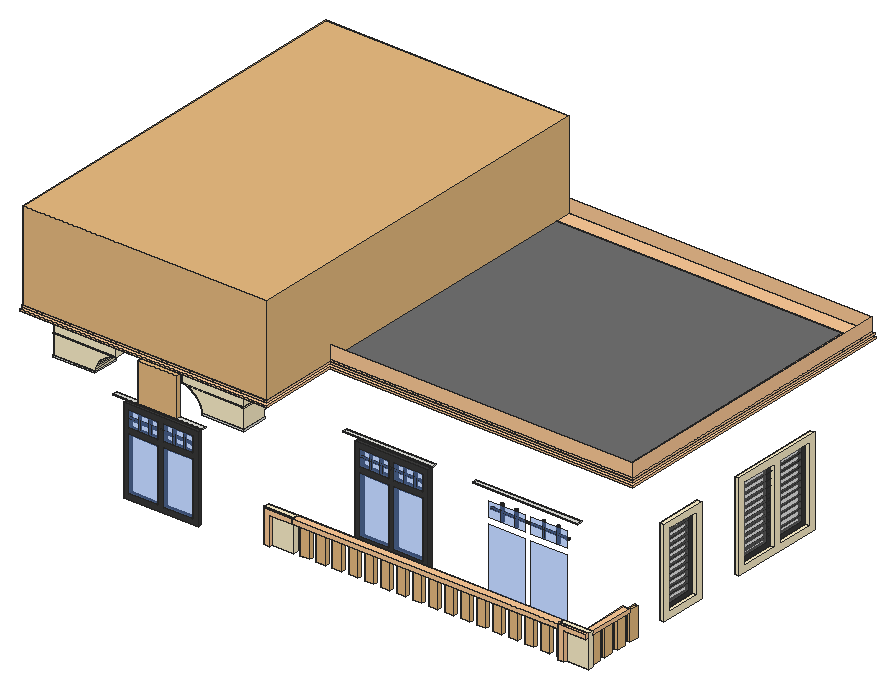
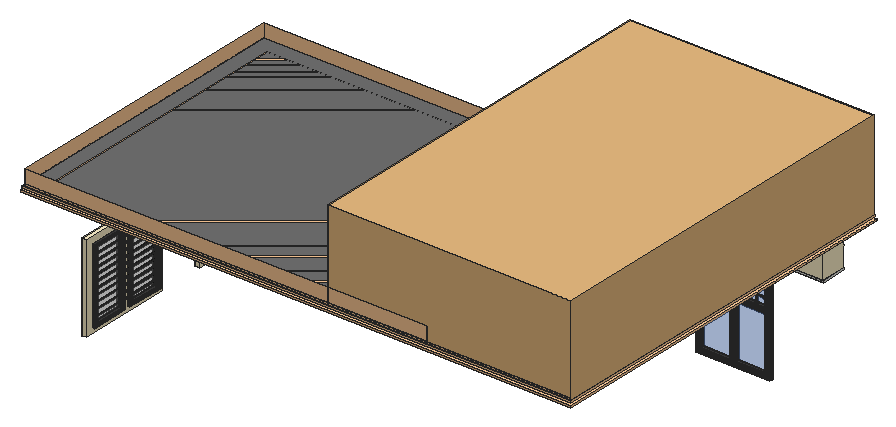
# SketchUp Ruby script. Lengths in inches.
U = 1.inch
M = Sketchup.active_model
def pt(a) = Geom::Point3d.new(a.map { |v| v * U })
def face(e, loops, mat)
  f = e.add_face(loops[0].map { |a| pt(a) })
  loops[1..].each { |l| e.add_face(l.map { |a| pt(a) }).erase! }
  f.material = f.back_material = mat if mat
  f
end
# faces: each face lists its corners as indices into pts; further lists are holes
def faces(e, pts, list, mat = nil) = list.each { |f| face(e, (f[0].is_a?(Array) ? f : [f]).map { |l| l.map { |i| pts[i] } }, mat) }
# xy, xz, yz: faces in a plane at the given z, y or x. An outline is a flat list of corners, or four numbers for a rectangle; further outlines are holes
def ring(l) = l.size == 4 ? [[l[0], l[1]], [l[2], l[1]], [l[2], l[3]], [l[0], l[3]]] : l.each_slice(2).to_a
def flat(e, list, mat, &to3) = list.each { |f| face(e, (f[0].is_a?(Array) ? f : [f]).map { |l| ring(l).map { |u, v| to3.(u, v) } }, mat) }
def xy(e, z, list, mat = nil) = flat(e, list, mat) { |x, y| [x, y, z] }
def xz(e, y, list, mat = nil) = flat(e, list, mat) { |x, z| [x, y, z] }
def yz(e, x, list, mat = nil) = flat(e, list, mat) { |y, z| [x, y, z] }
def lines(e, pts, list) = list.each { |a, b| e.add_line(pt(pts[a]), pt(pts[b])) }
# prism: a flat outline (further loops are holes) pulled along v
def prism(e, loops, v, mat = nil)
  f = face(e, loops, mat); d = Geom::Vector3d.new(v.map { |x| x * U })
  f.pushpull(f.normal.samedirection?(d) ? d.length : -d.length)
end
def box(e, o, s, mat = nil) = prism(e, [[o, [o[0] + s[0], o[1], o[2]], [o[0] + s[0], o[1] + s[1], o[2]], [o[0], o[1] + s[1], o[2]]]], [0, 0, s[2]], mat)
def at(x, y, z, deg = 0) = Geom::Transformation.translation(pt([x, y, z])) * Geom::Transformation.rotation(ORIGIN, Z_AXIS, deg.degrees)
def axes(o, x, y, z) = Geom::Transformation.new([*x, 0, *y, 0, *z, 0, *pt(o).to_a, 1])
def part(name) = M.definitions.add(name)
# library, detail: a bought-in or finely detailed component or shape, given as its bounding box
def library(name, o, s) = part(name).tap { |d| box(d.entities, o, s) }
def detail(e, o, s) = box(e.add_group.entities, o, s)
def put(e, d, t, mat = nil) = e.add_instance(d, t).tap { |i| i.material = mat if mat }
def group(e, t, mat = nil) = e.add_group.tap { |g| g.transformation = t; g.material = mat if mat }.entities
root = M.entities
M.materials.add("[Color C02]").color = [255, 204, 153]
M.materials.add("[Color D01]").color = [255, 242, 204]
M.materials.add("[Color M05]").color = [114, 114, 114]
M.materials.add("[Color M07]").color = [58, 58, 58]
M.materials.add("[Color M08]").color = [30, 30, 30]
M.materials.add("[Translucent Glass Blue]").color = [100, 149, 237]
M.materials["[Translucent Glass Blue]"].alpha = 0.5
M.materials.add("[Translucent Glass Gray]").color = [128, 128, 128]
M.materials["[Translucent Glass Gray]"].alpha = 0.5
c1 = part("Group\#116")
box(c1.entities,[0,0,0],[33.28,6,36])
c2 = part("Group\#117")
xy(c2.entities,0,[[0,0,7.19,3]])
xy(c2.entities,31.08,[[7.19,0,31.28,3]])
xy(c2.entities,36,[[0,0,7.19,3],[7.19,0,31.28,3]])
xz(c2.entities,0,[[0,0,7.19,0,7.19,31.08,31.28,31.08,31.28,36,0,36]])
xz(c2.entities,3,[[0,0,7.19,36],[7.19,31.08,31.28,36]])
yz(c2.entities,0,[[0,0,3,36]])
yz(c2.entities,7.19,[[0,0,3,31.08]])
yz(c2.entities,31.28,[[0,31.08,3,36]])
c3 = library("Group\#119",[0,0,0],[10.6875,3.6875,32.1875])
c4 = part("Group\#73")
prism(c4.entities,[[[0.41,0,0.11],[0.6,0,0.03],[0.8125,0,0],[1.02,0,0.03],[1.22,0,0.11],[1.39,0,0.24],[1.52,0,0.41],[1.6,0,0.6],[1.625,0,0.8125],[1.6,0,1.02],[1.52,0,1.22],[1.39,0,1.39],[1.22,0,1.52],[1.02,0,1.6],[0.8125,0,1.625],[0.6,0,1.6],[0.41,0,1.52],[0.24,0,1.39],[0.11,0,1.22],[0.03,0,1.02],[0,0,0.8125],[0.03,0,0.6],[0.11,0,0.41],[0.24,0,0.24]]],[0,83.52,0])
c5 = part("Group\#71")
prism(c5.entities,[[[1.26,30.72,0.03],[1,30.72,0],[0.74,30.72,0.03],[0.5,30.72,0.13],[0.29,30.72,0.29],[0.13,30.72,0.5],[0.03,30.72,0.74],[0,30.72,1],[0.03,30.72,1.26],[0.13,30.72,1.5],[0.29,30.72,1.71],[0.5,30.72,1.87],[0.74,30.72,1.97],[1,30.72,2],[1.26,30.72,1.97],[1.5,30.72,1.87],[1.71,30.72,1.71],[1.87,30.72,1.5],[1.97,30.72,1.26],[2,30.72,1],[1.97,30.72,0.74],[1.87,30.72,0.5],[1.71,30.72,0.29],[1.5,30.72,0.13]]],[0,-30.72,0])
c6 = part("Group\#104")
box(c6.entities,[-1,-1,0],[47.74,29,1.9375])
c7 = library("Group\#113",[-1.05,-1.3,0],[273.09,424.42,99.7])
xy(root,387.9375,[[446.12,288.64,786.76,619.71]])
xy(root,391.9375,[[338.37,286.64,788.76,621.71]],"[Color M05]")
xz(root,286.64,[[338.37,391.9375,788.76,407.09]],"[Color C02]")
xz(root,621.71,[[338.37,391.9375,788.76,407.09]],"[Color C02]")
yz(root,338.37,[[286.64,391.9375,621.71,407.09]],"[Color M05]")
yz(root,788.76,[[286.64,391.9375,621.71,407.09]],"[Color C02]")
g1 = group(root,at(660.76,304.14,204),"[Translucent Glass Blue]")
xz(g1,0,[[0,0,41,72]])
g2 = group(root,at(613.76,304.14,204),"[Translucent Glass Blue]")
xz(g2,0,[[0,0,41,72]])
g3 = group(root,at(462.04,304.64,206),"[Color M07]")
prism(g3,[[[82.52,5,0],[0,5,0],[0,5,100],[82.52,5,100]],[[6,5,6],[38.26,5,6],[38.26,5,70],[6,5,70]],[[44.26,5,70],[44.26,5,6],[76.52,5,6],[76.52,5,70]],[[6,5,76],[38.26,5,76],[38.26,5,94],[6,5,94]],[[44.26,5,76],[76.52,5,76],[76.52,5,94],[44.26,5,94]]],[0,-5,0])
g4 = group(root,at(260.38,232.64,210),"[Color M07]")
prism(g4,[[[0,0,96],[0,0,0],[84,0,0],[84,0,96]],[[6,0,66],[39,0,66],[39,0,6],[6,0,6]],[[78,0,66],[78,0,6],[45,0,6],[45,0,66]],[[78,0,72],[45,0,72],[45,0,90],[78,0,90]],[[6,0,72],[6,0,90],[39,0,90],[39,0,72]]],[0,4,0])
put(root,c1,at(406.12,247.64,210),"[Color D01]")
put(root,c2,at(408.12,244.64,210),"[Color C02]")
put(root,c1,at(737.48,247.64,210),"[Color D01]")
put(root,c2,at(738.31,244.64,210),"[Color C02]")
put(root,c3,at(445.87,248.72,210),"[Color D01]")
put(root,c3,at(463.87,248.72,210),"[Color D01]")
put(root,c3,at(481.87,248.72,210),"[Color D01]")
put(root,c3,at(499.87,248.72,210),"[Color D01]")
put(root,c3,at(517.87,248.72,210),"[Color D01]")
put(root,c3,at(535.87,248.72,210),"[Color D01]")
put(root,c3,at(553.87,248.72,210),"[Color D01]")
put(root,c3,at(571.87,248.72,210),"[Color D01]")
put(root,c3,at(589.87,248.72,210),"[Color D01]")
put(root,c3,at(607.87,248.72,210),"[Color D01]")
put(root,c3,at(625.87,248.72,210),"[Color D01]")
put(root,c3,at(643.87,248.72,210),"[Color D01]")
put(root,c3,at(661.87,248.72,210),"[Color D01]")
put(root,c3,at(679.87,248.72,210),"[Color D01]")
put(root,c3,at(697.87,248.72,210),"[Color D01]")
put(root,c3,at(715.87,248.72,210),"[Color D01]")
put(root,c3,at(733.87,248.72,210),"[Color D01]")
put(root,c3,at(768.73,254.28,210,90),"[Color D01]")
put(root,c3,at(768.73,272.28,210,90),"[Color D01]")
put(root,c3,at(768.73,290.28,210,90),"[Color D01]")
put(root,c3,at(768.73,308.28,210,90))
g5 = group(root,at(468.04,304.64,212),"[Translucent Glass Blue]")
xz(g5,0,[[0,0,32.26,64]])
g6 = group(root,at(506.3,304.64,212),"[Translucent Glass Blue]")
xz(g6,0,[[0,0,32.26,64]])
g7 = group(root,at(770.76,346.79,216),"[Color D01]")
prism(g7,[[[0,52.72,98],[0,52.72,0],[0,0,0],[0,0,98]],[[0,7,7],[0,45.72,7],[0,45.72,91],[0,7,91]]],[5,0,0])
g8 = group(root,at(770.76,452.39,216),"[Color D01]")
prism(g8,[[[0,0,98],[0,105.52,98],[0,105.52,0],[0,0,0]],[[0,7,91],[0,7,7],[0,49.26,7],[0,49.26,91]],[[0,98.52,91],[0,56.26,91],[0,56.26,7],[0,98.52,7]]],[5,0,0])
g9 = group(root,at(266.38,232.64,216),"[Translucent Glass Blue]")
xz(g9,0,[[0,0,33,60]])
g10 = group(root,at(305.38,232.64,216),"[Translucent Glass Blue]")
xz(g10,0,[[0,0,33,60]])
g11 = group(root,at(766.76,353.79,223),"[Color M07]")
prism(g11,[[[0,0,84],[0,38.72,84],[0,38.72,0],[0,0,0]],[[0,4,4],[0,34.72,4],[0,34.72,80],[0,4,80]]],[4,0,0])
g12 = group(root,at(766.76,459.39,223),"[Color M07]")
prism(g12,[[[0,0,84],[0,42.26,84],[0,42.26,0],[0,0,0]],[[0,38.26,4],[0,38.26,80],[0,4,80],[0,4,4]]],[4,0,0])
g13 = group(root,at(766.76,508.65,223),"[Color M07]")
prism(g13,[[[4,0,84],[4,0,0],[4,42.26,0],[4,42.26,84]],[[4,4,4],[4,4,80],[4,38.26,80],[4,38.26,4]]],[-4,0,0])
g14 = group(root,at(770.76,357.79,227),"[Translucent Glass Gray]")
yz(g14,0,[[0,0,30.72,76]])
g15 = group(root,at(770.76,512.65,227),"[Translucent Glass Gray]")
yz(g15,0,[[0,0,34.26,76]])
g16 = group(root,at(770.76,463.39,227),"[Translucent Glass Gray]")
yz(g16,0,[[0,0,34.26,76]])
put(root,c4,at(767.95,463.39,232.02),"[Color M08]")
put(root,c5,at(767.76,357.79,233.39),"[Color M08]")
put(root,c4,at(767.95,463.39,239.02),"[Color M08]")
put(root,c5,at(767.76,357.79,240.39),"[Color M08]")
g17 = group(root,at(439.4,244.64,241.08),"[Color C02]")
box(g17,[0,0,0],[298.91,9,4.92])
g18 = group(root,at(763.51,253.64,242),"[Color C02]")
box(g18,[0,0,0.1875],[7.25,51,3.8125])
put(root,c4,at(767.95,463.39,246.02),"[Color M08]")
put(root,c5,at(767.76,357.79,247.39),"[Color M08]")
put(root,c4,at(767.95,463.39,253.02),"[Color M08]")
put(root,c5,at(767.76,357.79,254.39),"[Color M08]")
put(root,c4,at(767.95,463.39,260.02),"[Color M08]")
put(root,c5,at(767.76,357.79,261.39),"[Color M08]")
put(root,c4,at(767.95,463.39,267.02),"[Color M08]")
put(root,c5,at(767.76,357.79,268.39),"[Color M08]")
put(root,c4,at(767.95,463.39,274.02),"[Color M08]")
put(root,c5,at(767.76,357.79,275.39),"[Color M08]")
put(root,c4,at(767.95,463.39,281.02),"[Color M08]")
g19 = group(root,at(625.26,305.64,282),"[Color M08]")
prism(g19,[[[1.26,1.96,0],[1.5,1.86,0],[1.71,1.7,0],[1.87,1.5,0],[1.97,1.25,0],[2,1,0],[1.96,0.74,0],[1.86,0.5,0],[1.7,0.29,0],[1.5,0.13,0],[1.25,0.03,0],[1,0,0],[0.74,0.04,0],[0.5,0.14,0],[0.29,0.3,0],[0.13,0.5,0],[0.03,0.75,0],[0,1,0],[0.04,1.26,0],[0.14,1.5,0],[0.3,1.71,0],[0.5,1.87,0],[0.75,1.97,0],[1,2,0]]],[0,0,18])
g20 = group(root,at(641.27,305.64,282),"[Color M08]")
prism(g20,[[[0.18,0.41,0],[0.06,0.64,0],[0,0.9,0],[0.01,1.16,0],[0.08,1.41,0],[0.22,1.63,0],[0.41,1.81,0],[0.64,1.93,0],[0.9,1.99,0],[1.16,1.98,0],[1.41,1.91,0],[1.63,1.77,0],[1.81,1.58,0],[1.93,1.35,0],[1.99,1.09,0],[1.98,0.83,0],[1.91,0.58,0],[1.77,0.36,0],[1.58,0.18,0],[1.35,0.06,0],[1.09,0,0],[0.83,0.01,0],[0.58,0.08,0],[0.36,0.22,0]]],[0,0,18])
g21 = group(root,at(672.26,305.64,282),"[Color M08]")
prism(g21,[[[0.03,0.74,0],[0,1,0],[0.03,1.26,0],[0.13,1.5,0],[0.29,1.71,0],[0.5,1.87,0],[0.74,1.97,0],[1,2,0],[1.26,1.97,0],[1.5,1.87,0],[1.71,1.71,0],[1.87,1.5,0],[1.97,1.26,0],[2,1,0],[1.97,0.74,0],[1.87,0.5,0],[1.71,0.29,0],[1.5,0.13,0],[1.26,0.03,0],[1,0,0],[0.74,0.03,0],[0.5,0.13,0],[0.29,0.29,0],[0.13,0.5,0]]],[0,0,18])
g22 = group(root,at(688.27,305.64,282),"[Color M08]")
prism(g22,[[[1.99,1.11,0],[1.98,0.85,0],[1.91,0.6,0],[1.78,0.37,0],[1.59,0.19,0],[1.36,0.0625,0],[1.11,0,0],[0.85,0,0],[0.6,0.08,0],[0.37,0.21,0],[0.19,0.4,0],[0.0625,0.625,0],[0,0.88,0],[0,1.14,0],[0.08,1.39,0],[0.21,1.61,0],[0.4,1.8,0],[0.625,1.92,0],[0.88,1.99,0],[1.14,1.98,0],[1.39,1.91,0],[1.61,1.78,0],[1.8,1.59,0],[1.92,1.36,0]]],[0,0,18])
g23 = group(root,at(613.76,304.14,282),"[Translucent Glass Blue]")
xz(g23,0,[[0,0,41,18]])
g24 = group(root,at(660.76,304.14,282),"[Translucent Glass Blue]")
xz(g24,0,[[0,0,41,18]])
g25 = group(root,at(489.17,306.14,282),"[Color M08]")
prism(g25,[[[1,0,0],[0.74,0.03,0],[0.5,0.13,0],[0.29,0.29,0],[0.13,0.5,0],[0.03,0.74,0],[0,1,0],[0.03,1.26,0],[0.13,1.5,0],[0.29,1.71,0],[0.5,1.87,0],[0.74,1.97,0],[1,2,0],[1.26,1.97,0],[1.5,1.87,0],[1.71,1.71,0],[1.87,1.5,0],[1.97,1.26,0],[2,1,0],[1.97,0.74,0],[1.87,0.5,0],[1.71,0.29,0],[1.5,0.13,0],[1.26,0.03,0]]],[0,0,18])
g26 = group(root,at(477.17,306.14,282),"[Color M08]")
prism(g26,[[[0.13,1.5,0],[0.29,1.71,0],[0.5,1.87,0],[0.74,1.97,0],[1,2,0],[1.26,1.97,0],[1.5,1.87,0],[1.71,1.71,0],[1.87,1.5,0],[1.97,1.26,0],[2,1,0],[1.97,0.74,0],[1.87,0.5,0],[1.71,0.29,0],[1.5,0.13,0],[1.26,0.03,0],[1,0,0],[0.74,0.03,0],[0.5,0.13,0],[0.29,0.29,0],[0.13,0.5,0],[0.03,0.74,0],[0,1,0],[0.03,1.26,0]]],[0,0,18])
g27 = group(root,at(527.43,306.14,282),"[Color M08]")
prism(g27,[[[0.03,1.26,0],[0.13,1.5,0],[0.29,1.71,0],[0.5,1.87,0],[0.74,1.97,0],[1,2,0],[1.26,1.97,0],[1.5,1.87,0],[1.71,1.71,0],[1.87,1.5,0],[1.97,1.26,0],[2,1,0],[1.97,0.74,0],[1.87,0.5,0],[1.71,0.29,0],[1.5,0.13,0],[1.26,0.03,0],[1,0,0],[0.74,0.03,0],[0.5,0.13,0],[0.29,0.29,0],[0.13,0.5,0],[0.03,0.74,0],[0,1,0]]],[0,0,18.0625])
g28 = group(root,at(515.4375,306.14,282),"[Color M08]")
prism(g28,[[[0.03,1.25,0],[0.13,1.5,0],[0.29,1.7,0],[0.5,1.86,0],[0.74,1.96,0],[1,1.99,0],[1.25,1.96,0],[1.5,1.86,0],[1.7,1.7,0],[1.86,1.5,0],[1.96,1.25,0],[1.99,1,0],[1.96,0.74,0],[1.86,0.5,0],[1.7,0.29,0],[1.5,0.13,0],[1.25,0.03,0],[1,0,0],[0.74,0.03,0],[0.5,0.13,0],[0.29,0.29,0],[0.13,0.5,0],[0.03,0.74,0],[0,1,0]]],[0,0,18])
g29 = group(root,at(468.04,304.64,282),"[Translucent Glass Blue]")
xz(g29,0,[[0,0,32.26,18]])
g30 = group(root,at(506.3,304.64,282),"[Translucent Glass Blue]")
xz(g30,0,[[0,0,32.26,18]])
g31 = group(root,at(275.88,233.64,282),"[Color M08]")
prism(g31,[[[1.97,0.74,0],[1.87,0.5,0],[1.71,0.29,0],[1.5,0.13,0],[1.26,0.03,0],[1,0,0],[0.74,0.03,0],[0.5,0.13,0],[0.29,0.29,0],[0.13,0.5,0],[0.03,0.74,0],[0,1,0],[0.03,1.26,0],[0.13,1.5,0],[0.29,1.71,0],[0.5,1.87,0],[0.74,1.97,0],[1,2,0],[1.26,1.97,0],[1.5,1.87,0],[1.71,1.71,0],[1.87,1.5,0],[1.97,1.26,0],[2,1,0]]],[0,0,18])
g32 = group(root,at(287.88,233.64,282),"[Color M08]")
prism(g32,[[[2,1,0],[1.97,0.74,0],[1.87,0.5,0],[1.71,0.29,0],[1.5,0.13,0],[1.26,0.03,0],[1,0,0],[0.74,0.03,0],[0.5,0.13,0],[0.29,0.29,0],[0.13,0.5,0],[0.03,0.74,0],[0,1,0],[0.03,1.26,0],[0.13,1.5,0],[0.29,1.71,0],[0.5,1.87,0],[0.74,1.97,0],[1,2,0],[1.26,1.97,0],[1.5,1.87,0],[1.71,1.71,0],[1.87,1.5,0],[1.97,1.26,0]]],[0,0,18])
g33 = group(root,at(314.88,233.64,282),"[Color M08]")
prism(g33,[[[1,0,0],[0.74,0.03,0],[0.5,0.13,0],[0.29,0.29,0],[0.13,0.5,0],[0.03,0.74,0],[0,1,0],[0.03,1.26,0],[0.13,1.5,0],[0.29,1.71,0],[0.5,1.87,0],[0.74,1.97,0],[1,2,0],[1.26,1.97,0],[1.5,1.87,0],[1.71,1.71,0],[1.87,1.5,0],[1.97,1.26,0],[2,1,0],[1.97,0.74,0],[1.87,0.5,0],[1.71,0.29,0],[1.5,0.13,0],[1.26,0.03,0]]],[0,0,18])
g34 = group(root,at(326.88,233.64,282),"[Color M08]")
prism(g34,[[[1.71,1.71,0],[1.87,1.5,0],[1.97,1.26,0],[2,1,0],[1.97,0.74,0],[1.87,0.5,0],[1.71,0.29,0],[1.5,0.13,0],[1.26,0.03,0],[1,0,0],[0.74,0.03,0],[0.5,0.13,0],[0.29,0.29,0],[0.13,0.5,0],[0.03,0.74,0],[0,1,0],[0.03,1.26,0],[0.13,1.5,0],[0.29,1.71,0],[0.5,1.87,0],[0.74,1.97,0],[1,2,0],[1.26,1.97,0],[1.5,1.87,0]]],[0,0,18])
g35 = group(root,at(266.38,232.64,282),"[Translucent Glass Blue]")
xz(g35,0,[[0,0,33,18]])
g36 = group(root,at(305.38,232.64,282),"[Translucent Glass Blue]")
xz(g36,0,[[0,0,33,18]])
put(root,c5,at(767.76,357.79,282.39),"[Color M08]")
put(root,c4,at(767.95,463.39,288.02),"[Color M08]")
put(root,c5,at(767.76,357.79,289.39),"[Color M08]")
g37 = group(root,at(613.76,305.64,290),"[Color M08]")
prism(g37,[[[88,0.74,0.03],[88,1,0],[88,1.26,0.03],[88,1.5,0.13],[88,1.71,0.29],[88,1.87,0.5],[88,1.97,0.74],[88,2,1],[88,1.97,1.26],[88,1.87,1.5],[88,1.71,1.71],[88,1.5,1.87],[88,1.26,1.97],[88,1,2],[88,0.74,1.97],[88,0.5,1.87],[88,0.29,1.71],[88,0.13,1.5],[88,0.03,1.26],[88,0,1],[88,0.03,0.74],[88,0.13,0.5],[88,0.29,0.29],[88,0.5,0.13]]],[-88,0,0])
g38 = group(root,at(468.04,306.14,290),"[Color M08]")
prism(g38,[[[70.52,0.74,0.03],[70.52,1,0],[70.52,1.26,0.03],[70.52,1.5,0.13],[70.52,1.71,0.29],[70.52,1.87,0.5],[70.52,1.97,0.74],[70.52,2,1],[70.52,1.97,1.26],[70.52,1.87,1.5],[70.52,1.71,1.71],[70.52,1.5,1.87],[70.52,1.26,1.97],[70.52,1,2],[70.52,0.74,1.97],[70.52,0.5,1.87],[70.52,0.29,1.71],[70.52,0.13,1.5],[70.52,0.03,1.26],[70.52,0,1],[70.52,0.03,0.74],[70.52,0.13,0.5],[70.52,0.29,0.29],[70.52,0.5,0.13]]],[-70.52,0,0])
g39 = group(root,at(266.38,233.64,290),"[Color M08]")
prism(g39,[[[0,1,0],[0,0.74,0.03],[0,0.5,0.13],[0,0.29,0.29],[0,0.13,0.5],[0,0.03,0.74],[0,0,1],[0,0.03,1.26],[0,0.13,1.5],[0,0.29,1.71],[0,0.5,1.87],[0,0.74,1.97],[0,1,2],[0,1.26,1.97],[0,1.5,1.87],[0,1.71,1.71],[0,1.87,1.5],[0,1.97,1.26],[0,2,1],[0,1.97,0.74],[0,1.87,0.5],[0,1.71,0.29],[0,1.5,0.13],[0,1.26,0.03]]],[72,0,0])
put(root,c4,at(767.95,463.39,295.02),"[Color M08]")
put(root,c5,at(767.76,357.79,296.39),"[Color M08]")
g40 = group(root,at(252.38,227.64,313))
box(g40,[0,0,0],[100,5,1])
g41 = group(root,at(598.76,299.64,314))
box(g41,[0,0,0],[118,5,1])
g42 = group(root,at(453.04,299.64,314))
box(g42,[0,0,0],[100.52,5,1])
g43 = group(root,at(280.72,227.64,314),"[Translucent Glass Gray]")
detail(g43,[0,0,0],[43.33,5,43.33])
put(root,c6,at(362.38,216.64,336))
put(root,c6,at(195.13,216.64,336))
g44 = group(root,at(362.38,216.64,337.9375),"[Color D01]")
xy(g44,0,[[-1,0,45.74,28]])
xy(g44,22.0625,[[45.74,0,46.74,46]])
xy(g44,22.5625,[[45.74,0,46.74,46]])
xy(g44,36,[[-24,0,45.74,0,45.74,46,36,46,36,28,-24,28]])
xz(g44,0,[[-1,0,45.74,0,45.74,22.0625,46.74,22.0625,46.74,22.5625,45.74,22.5625,45.74,36,-24,36,-24,22.0625,-21.17,21.62,-18.41,20.87,-15.75,19.82,-13.23,18.47,-10.86,16.86,-8.69,15,-6.74,12.91,-5.03,10.61,-3.59,8.15,-2.43,5.53,-1.56,2.81]])
xz(g44,28,[[-1,0,-1.56,2.81,-2.43,5.53,-3.59,8.15,-5.03,10.61,-6.74,12.91,-8.69,15,-10.86,16.86,-13.23,18.47,-15.75,19.82,-18.41,20.87,-21.17,21.62,-24,22.0625,-24,36,36,36,36,0]])
xz(g44,46,[[36,22.0625,36,36,45.74,36,45.74,22.5625,46.74,22.5625,46.74,22.0625]])
yz(g44,-24,[[0,22.0625,28,36]])
yz(g44,36,[[28,0,28,34.9375,46,34.9375,46,22.0625,43.46,21.52,41,20.67,38.66,19.52,36.49,18.1,34.5,16.42,32.74,14.51,31.22,12.4,29.97,10.11,29.02,7.7,28.36,5.18,28.02,2.6],[28,34.9375,46,36]])
yz(g44,45.74,[[0,0,28,0,28.02,2.6,28.36,5.18,29.02,7.7,29.97,10.11,31.22,12.4,32.74,14.51,34.5,16.42,36.49,18.1,38.66,19.52,41,20.67,43.46,21.52,46,22.0625,0,22.0625],[0,22.5625,46,36]])
yz(g44,46.74,[[0,22.0625,46,22.5625]])
p = [[-1,0,0],[-1.56,0,2.81],[-1.56,28,2.81],[-1,28,0],[45.74,28.02,2.6],[45.74,28,0],
  [36,28,0],[36,28.02,2.6],[45.74,28.36,5.18],[36,28.36,5.18],[-2.43,0,5.53],[-2.43,28,5.53],
  [45.74,29.02,7.7],[36,29.02,7.7],[-3.59,0,8.15],[-3.59,28,8.15],[45.74,29.97,10.11],[36,29.97,10.11],
  [-5.03,0,10.61],[-5.03,28,10.61],[45.74,31.22,12.4],[36,31.22,12.4],[-6.74,0,12.91],[-6.74,28,12.91],
  [45.74,32.74,14.51],[36,32.74,14.51],[-8.69,0,15],[-8.69,28,15],[45.74,34.5,16.42],[36,34.5,16.42],
  [-10.86,0,16.86],[-10.86,28,16.86],[45.74,36.49,18.1],[36,36.49,18.1],[-13.23,0,18.47],[-13.23,28,18.47],
  [45.74,38.66,19.52],[36,38.66,19.52],[-15.75,0,19.82],[-15.75,28,19.82],[45.74,41,20.67],[36,41,20.67],
  [-18.41,0,20.87],[-18.41,28,20.87],[45.74,43.46,21.52],[36,43.46,21.52],[-21.17,0,21.62],[-21.17,28,21.62],
  [45.74,46,22.0625],[36,46,22.0625],[-24,0,22.0625],[-24,28,22.0625]]
faces(g44,p,[[0,1,2,3],[4,5,6,7],[8,4,7,9],[1,10,11,2],[12,8,9,13],[10,14,15,11],[16,12,13,17],[14,18,19,15],
  [20,16,17,21],[18,22,23,19],[24,20,21,25],[22,26,27,23],[28,24,25,29],[26,30,31,27],[32,28,29,33],[30,34,35,31],
  [36,32,33,37],[34,38,39,35],[40,36,37,41],[38,42,43,39],[44,40,41,45],[42,46,47,43],[48,44,45,49],[46,50,51,47]])
g45 = group(root,at(195.13,216.64,337.9375),"[Color D01]")
box(g45,[143.25,-1,22.0625],[70.74,1,0.5])
xy(g45,0,[[0,0,46.74,28]])
xy(g45,22.0625,[[0,-1,69.74,0]])
xy(g45,22.5625,[[0,-1,69.74,0]])
xy(g45,36,[[0,0,69.74,28]])
xz(g45,-1,[[0,22.0625,69.74,22.5625]])
xz(g45,0,[[0,0,46.74,0,47.3,2.81,48.17,5.53,49.33,8.15,50.77,10.61,52.48,12.91,54.43,15,56.6,16.86,58.97,18.47,61.49,19.82,64.15,20.87,66.91,21.62,69.74,22.0625,0,22.0625],[0,22.5625,69.74,36]])
xz(g45,28,[[0,0,0,36,69.74,36,69.74,22.0625,66.91,21.62,64.15,20.87,61.49,19.82,58.97,18.47,56.6,16.86,54.43,15,52.48,12.91,50.77,10.61,49.33,8.15,48.17,5.53,47.3,2.81,46.74,0]])
yz(g45,0,[[0,0,0,22.0625,-1,22.0625,-1,22.5625,0,22.5625,0,36,28,36,28,0]])
yz(g45,69.74,[[-1,22.0625,28,22.0625,28,36,0,36,0,22.5625,-1,22.5625]])
p = [[47.3,0,2.81],[46.74,0,0],[46.74,28,0],[47.3,28,2.81],[48.17,0,5.53],[48.17,28,5.53],
  [49.33,0,8.15],[49.33,28,8.15],[50.77,0,10.61],[50.77,28,10.61],[52.48,0,12.91],[52.48,28,12.91],
  [54.43,0,15],[54.43,28,15],[56.6,0,16.86],[56.6,28,16.86],[58.97,0,18.47],[58.97,28,18.47],
  [61.49,0,19.82],[61.49,28,19.82],[64.15,0,20.87],[64.15,28,20.87],[66.91,0,21.62],[66.91,28,21.62],
  [69.74,0,22.0625],[69.74,28,22.0625]]
faces(g45,p,[[0,1,2,3],[4,0,3,5],[6,4,5,7],[8,6,7,9],[10,8,9,11],[12,10,11,13],[14,12,13,15],[16,14,15,17],
  [18,16,17,19],[20,18,19,21],[22,20,21,23],[24,22,23,25]])
g46 = group(root,at(195.13,216.64,373.9375),"[Color C02]")
prism(g46,[[[575.63,88,-3.6875],[234.99,88,-3.6875],[234.99,0,-3.6875],[0,0,-3.6875],[0,387.07,-3.6875],[575.63,387.07,-3.6875]]],[0,0,21.6875])
g47 = group(root,at(174.13,195.64,373.9375),"[Color C02]")
xy(g47,0,[[[17,17,17,412.07,600.63,412.07,600.63,105,259.99,105,259.99,17],[21,21,255.99,21,255.99,109,596.63,109,596.63,408.07,21,408.07]]])
xy(g47,2,[[[17,17,259.99,17,259.99,105,600.63,105,600.63,412.07,17,412.07],[19,19,19,410.07,598.63,410.07,598.63,107,257.99,107,257.99,19]]])
xy(g47,4,[[[13,13,13,416.07,604.63,416.07,604.63,101,263.99,101,263.99,13],[19,19,257.99,19,257.99,107,598.63,107,598.63,410.07,19,410.07]]])
xy(g47,6,[[[13,13,263.99,13,263.99,101,604.63,101,604.63,416.07,13,416.07],[16,16,16,413.07,601.63,413.07,601.63,104,260.99,104,260.99,16]]])
xy(g47,9,[[21,21,21,408.07,596.63,408.07,596.63,109,255.99,109,255.99,21]])
xy(g47,10,[[[0,0,0,429.07,617.63,429.07,617.63,88,276.99,88,276.99,0],[16,16,260.99,16,260.99,104,601.63,104,601.63,413.07,16,413.07]]])
xy(g47,12,[[[0,0,276.99,0,276.99,88,617.63,88,617.63,429.07,0,429.07],[5,5,5,424.07,612.63,424.07,612.63,93,271.99,93,271.99,5]]])
xy(g47,14,[[[1,1,1,428.07,616.63,428.07,616.63,89,275.99,89,275.99,1],[5,5,271.99,5,271.99,93,612.63,93,612.63,424.07,5,424.07]]])
xy(g47,16,[[[1,1,275.99,1,275.99,89,616.63,89,616.63,428.07,1,428.07],[3,3,3,426.07,614.63,426.07,614.63,91,273.99,91,273.99,3]]])
xy(g47,18,[[[3,3,273.99,3,273.99,91,614.63,91,614.63,426.07,3,426.07],[21,21,21,408.07,596.63,408.07,596.63,109,255.99,109,255.99,21]]])
xz(g47,0,[[0,10,276.99,12]])
xz(g47,1,[[1,14,275.99,16]])
xz(g47,3,[[3,16,273.99,18]])
xz(g47,5,[[5,12,271.99,14]])
xz(g47,13,[[13,4,263.99,6]])
xz(g47,16,[[16,6,260.99,10]])
xz(g47,17,[[17,0,259.99,2]])
xz(g47,19,[[19,2,257.99,4]])
xz(g47,21,[[21,0,255.99,9],[21,9,255.99,18]])
xz(g47,88,[[276.99,10,617.63,12]])
xz(g47,89,[[275.99,14,616.63,16]])
xz(g47,91,[[273.99,16,614.63,18]])
xz(g47,93,[[271.99,12,612.63,14]])
xz(g47,101,[[263.99,4,604.63,6]])
xz(g47,104,[[260.99,6,601.63,10]])
xz(g47,105,[[259.99,0,600.63,2]])
xz(g47,107,[[257.99,2,598.63,4]])
xz(g47,109,[[255.99,0,596.63,9],[255.99,9,596.63,18]])
xz(g47,408.07,[[21,0,596.63,9],[21,9,596.63,18]])
xz(g47,410.07,[[19,2,598.63,4]])
xz(g47,412.07,[[17,0,600.63,2]])
xz(g47,413.07,[[16,6,601.63,10]])
xz(g47,416.07,[[13,4,604.63,6]])
xz(g47,424.07,[[5,12,612.63,14]])
xz(g47,426.07,[[3,16,614.63,18]])
xz(g47,428.07,[[1,14,616.63,16]])
xz(g47,429.07,[[0,10,617.63,12]])
yz(g47,0,[[0,10,429.07,12]])
yz(g47,1,[[1,14,428.07,16]])
yz(g47,3,[[3,16,426.07,18]])
yz(g47,5,[[5,12,424.07,14]])
yz(g47,13,[[13,4,416.07,6]])
yz(g47,16,[[16,6,413.07,10]])
yz(g47,17,[[17,0,412.07,2]])
yz(g47,19,[[19,2,410.07,4]])
yz(g47,21,[[21,0,408.07,9],[21,9,408.07,18]])
yz(g47,255.99,[[21,0,109,9],[21,9,109,18]])
yz(g47,257.99,[[19,2,107,4]])
yz(g47,259.99,[[17,0,105,2]])
yz(g47,260.99,[[16,6,104,10]])
yz(g47,263.99,[[13,4,101,6]])
yz(g47,271.99,[[5,12,93,14]])
yz(g47,273.99,[[3,16,91,18]])
yz(g47,275.99,[[1,14,89,16]])
yz(g47,276.99,[[0,10,88,12]])
yz(g47,596.63,[[109,0,408.07,9],[109,9,408.07,18]])
yz(g47,598.63,[[107,2,410.07,4]])
yz(g47,600.63,[[105,0,412.07,2]])
yz(g47,601.63,[[104,6,413.07,10]])
yz(g47,604.63,[[101,4,416.07,6]])
yz(g47,612.63,[[93,12,424.07,14]])
yz(g47,614.63,[[91,16,426.07,18]])
yz(g47,616.63,[[89,14,428.07,16]])
yz(g47,617.63,[[88,10,429.07,12]])
put(root,c7,at(177.13,198.58,389.9375),"[Color M05]")
